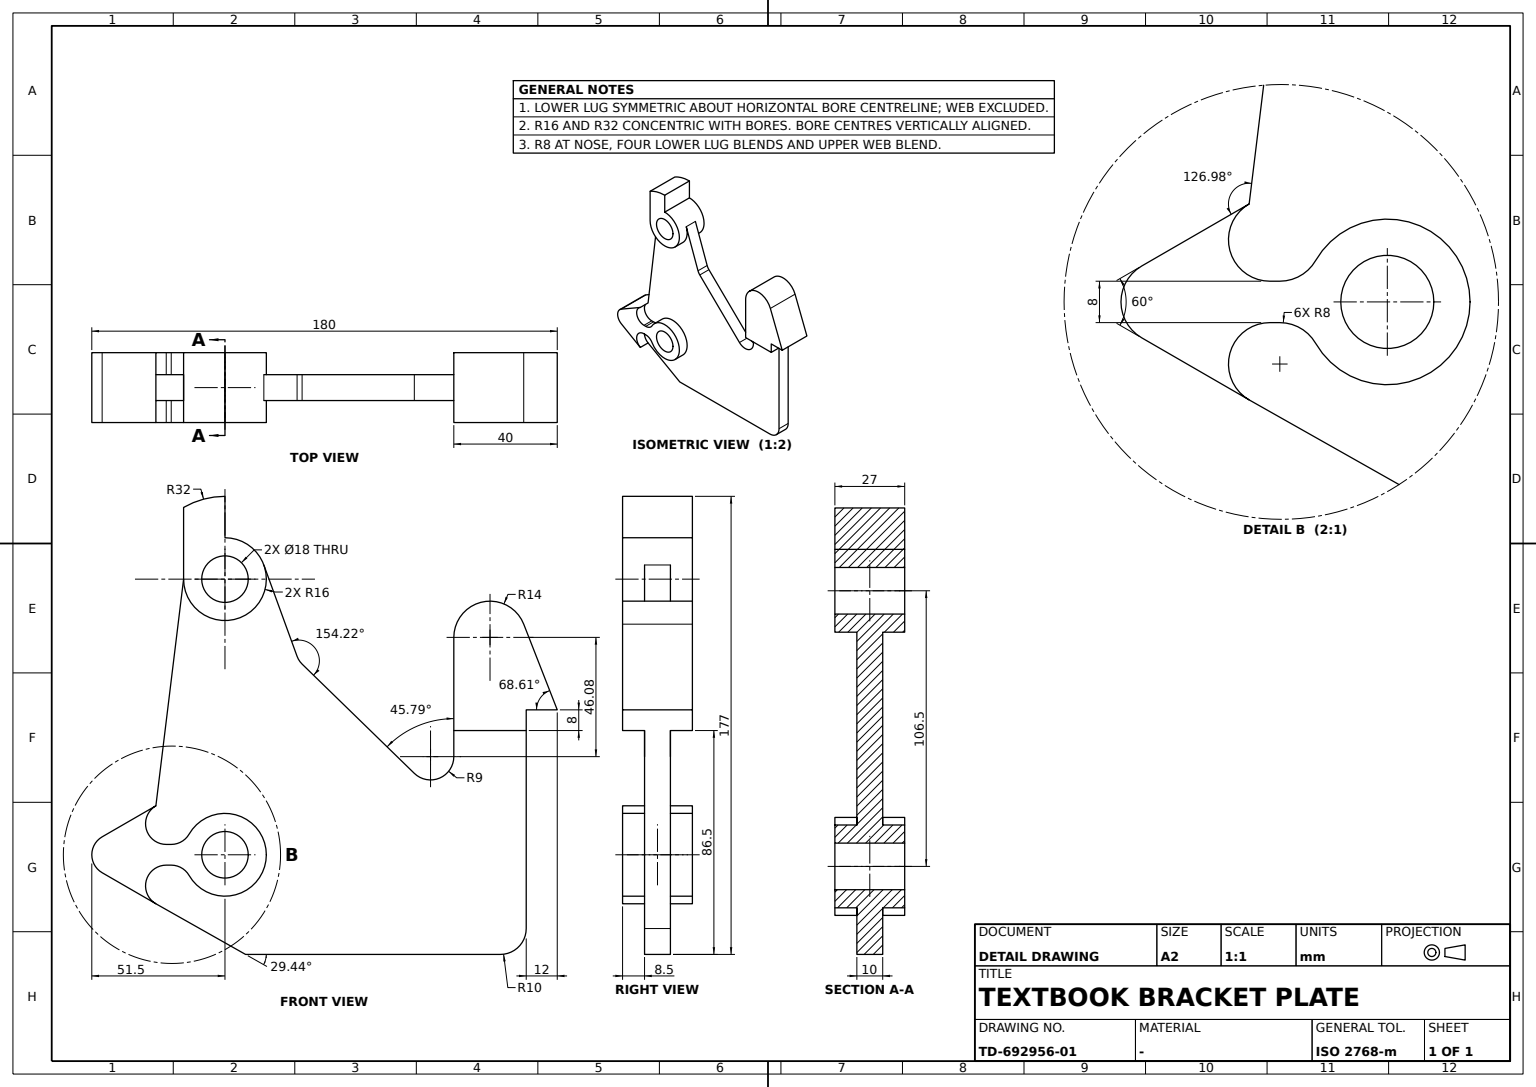
solid
v1 (-13.5,-26.71539,-18.928203)
v2 (-13.5,-22.71539,-4)
e1 v1 v2 CIRCLE(AX(P(-13.5,-22.71539,-12),D(-1,0,0),D(0,1,0)),8)
v3 (-5,-22.71539,-4)
e2 v2 v3 LINE
v4 (-5,-26.71539,-18.928203)
e3 v3 v4 CIRCLE(AX(P(-5,-22.71539,-12),D(1,0,0),D(0,1,0)),8)
e4 v1 v4 LINE
face CYL(AX(P(0,-22.71539,-12),D(-1,0,0),D(0,1,0)),8) rev [e1 e2 e3 -e4]
v5 (-5,106.5,-38.5)
v6 (-5,116.5,-28.5)
e5 v5 v6 CIRCLE(AX(P(-5,106.5,-28.5),D(1,0,0),D(0,1,0)),10)
v7 (5,116.5,-28.5)
e6 v6 v7 LINE
v8 (5,106.5,-38.5)
e7 v8 v7 CIRCLE(AX(P(5,106.5,-28.5),D(1,0,0),D(0,1,0)),10)
e8 v5 v8 LINE
face CYL(AX(P(0,106.5,-28.5),D(-1,0,0),D(0,1,0)),10) [e5 e6 -e7 -e8]
v9 (-5,16,106.5)
v10 (-13.5,16,106.5)
e9 v9 v10 LINE
v11 (-5,-16,106.5)
e10 v9 v11 CIRCLE(AX(P(-5,0,106.5),D(-1,0,0),D(0,1,0)),16)
v12 (-13.5,-16,106.5)
e11 v12 v11 LINE
e12 v12 v10 CIRCLE(AX(P(-13.5,0,106.5),D(1,0,0),D(0,1,0)),16)
face CYL(AX(P(0,0,106.5),D(-1,0,0),D(0,1,0)),16) [-e9 e10 -e11 e12]
v13 (-5,16,0)
v14 (-13.5,16,0)
e13 v13 v14 LINE
v15 (-5,-13.856406,-8)
e14 v13 v15 CIRCLE(AX(P(-5,0,0),D(-1,0,0),D(0,1,0)),16)
v16 (-13.5,-13.856406,-8)
e15 v16 v15 LINE
e16 v16 v14 CIRCLE(AX(P(-13.5,0,0),D(1,0,0),D(0,1,0)),16)
face CYL(AX(P(0,0,0),D(-1,0,0),D(0,1,0)),16) [-e13 e14 -e15 e16]
v17 (-13.5,9,0)
v18 (-13.5,-9,0)
e17 v17 v18 CIRCLE(AX(P(-13.5,0,0),D(1,0,0),D(0,1,0)),9)
v19 (13.5,9,0)
e18 v17 v19 LINE
v20 (13.5,-9,0)
e19 v19 v20 CIRCLE(AX(P(13.5,0,0),D(1,0,0),D(0,1,0)),9)
e20 v18 v20 LINE
face CYL(AX(P(0,0,0),D(-1,0,0),D(0,1,0)),9) rev [-e17 e18 e19 -e20]
v21 (13.5,16,0)
v22 (13.5,-13.856406,8)
e21 v21 v22 CIRCLE(AX(P(13.5,0,0),D(1,0,0),D(0,1,0)),16)
v23 (5,16,0)
e22 v21 v23 LINE
v24 (5,-13.856406,8)
e23 v24 v23 CIRCLE(AX(P(5,0,0),D(-1,0,0),D(0,1,0)),16)
e24 v24 v22 LINE
face CYL(AX(P(0,0,0),D(-1,0,0),D(0,1,0)),16) [-e21 e22 -e23 e24]
e25 v18 v17 CIRCLE(AX(P(-13.5,0,0),D(1,0,0),D(0,1,0)),9)
e26 v20 v19 CIRCLE(AX(P(13.5,0,0),D(1,0,0),D(0,1,0)),9)
face CYL(AX(P(0,0,0),D(-1,0,0),D(0,1,0)),9) rev [-e25 e20 e26 -e18]
v25 (-13.5,-26.71539,18.928203)
v26 (-5,-26.71539,18.928203)
e27 v25 v26 LINE
v27 (-13.5,-47.5,6.928203)
e28 v25 v27 LINE
v28 (13.5,-47.5,6.928203)
e29 v27 v28 LINE
v29 (13.5,-26.71539,18.928203)
e30 v29 v28 LINE
v30 (5,-26.71539,18.928203)
e31 v30 v29 LINE
e32 v26 v30 LINE
face PLANE(AX(P(0,-47.5,6.928203),D(0,0.5,-0.866025404),D(0,0.866025404,0.5))) rev [-e27 e28 e29 -e30 -e31 -e32]
v31 (-13.5,-47.5,-6.928203)
e33 v31 v1 LINE
v32 (5,-26.71539,-18.928203)
e34 v4 v32 LINE
v33 (13.5,-26.71539,-18.928203)
e35 v32 v33 LINE
v34 (13.5,-47.5,-6.928203)
e36 v34 v33 LINE
e37 v31 v34 LINE
face PLANE(AX(P(0,-47.5,-6.928203),D(0,-0.5,-0.866025404),D(0,0.866025404,-0.5))) [e33 e4 e34 e35 -e36 -e37]
v35 (5,-16,106.5)
e38 v35 v30 LINE
e39 v11 v35 LINE
e40 v11 v26 LINE
face PLANE(AX(P(0,-16,106.5),D(0,-0.992596896,0.121455349),D(0,-0.121455349,-0.992596896))) [e32 -e38 -e39 e40]
v36 (13.5,-13.856406,-8)
e41 v36 v21 CIRCLE(AX(P(13.5,0,0),D(1,0,0),D(0,1,0)),16)
v37 (5,-13.856406,-8)
e42 v37 v36 LINE
e43 v23 v37 CIRCLE(AX(P(5,0,0),D(-1,0,0),D(0,1,0)),16)
face CYL(AX(P(0,0,0),D(-1,0,0),D(0,1,0)),16) [-e22 -e41 -e42 -e43]
v38 (-5,116.5,48)
v39 (-5,88.5,48)
e44 v38 v39 LINE
v40 (-13.5,88.5,48)
e45 v40 v39 LINE
v41 (-13.5,116.5,48)
e46 v40 v41 LINE
e47 v41 v38 LINE
face PLANE(AX(P(0,88.5,48),D(0,0,-1),D(0,1,0))) [e44 -e45 e46 e47]
v42 (-5,27.888465,76.67917)
v43 (-5,15.034024,111.975228)
e48 v42 v43 LINE
v44 (5,15.034024,111.975228)
e49 v43 v44 LINE
v45 (5,27.888465,76.67917)
e50 v45 v44 LINE
e51 v42 v45 LINE
face PLANE(AX(P(0,27.888465,76.67917),D(0,0.9396265,0.342201754),D(0,-0.342201754,0.9396265))) [e48 e49 -e50 -e51]
v46 (-13.5,116.5,56)
v47 (13.5,116.5,56)
e52 v46 v47 LINE
v48 (-13.5,128.5,56)
e53 v46 v48 LINE
v49 (13.5,128.5,56)
e54 v48 v49 LINE
e55 v47 v49 LINE
face PLANE(AX(P(0,116.5,56),D(0,0,-1),D(0,1,0))) [-e52 e53 e54 -e55]
v50 (13.5,-20.78461,-4)
e56 v50 v36 CIRCLE(AX(P(13.5,-20.78461,-12),D(-1,0,0),D(0,1,0)),8)
v51 (5,-20.78461,-4)
e57 v51 v50 LINE
e58 v37 v51 CIRCLE(AX(P(5,-20.78461,-12),D(1,0,0),D(0,1,0)),8)
face CYL(AX(P(0,-20.78461,-12),D(-1,0,0),D(0,1,0)),8) rev [-e56 -e57 -e58 e42]
v52 (13.5,16,106.5)
v53 (5,16,106.5)
e59 v52 v53 LINE
v54 (13.5,-16,106.5)
e60 v54 v52 CIRCLE(AX(P(13.5,0,106.5),D(1,0,0),D(0,1,0)),16)
e61 v35 v54 LINE
e62 v53 v35 CIRCLE(AX(P(5,0,106.5),D(-1,0,0),D(0,1,0)),16)
face CYL(AX(P(0,0,106.5),D(-1,0,0),D(0,1,0)),16) [-e59 -e60 -e61 -e62]
v55 (-13.5,9,106.5)
v56 (-13.5,-9,106.5)
e63 v55 v56 CIRCLE(AX(P(-13.5,0,106.5),D(1,0,0),D(0,1,0)),9)
v57 (13.5,9,106.5)
e64 v55 v57 LINE
v58 (13.5,-9,106.5)
e65 v57 v58 CIRCLE(AX(P(13.5,0,106.5),D(1,0,0),D(0,1,0)),9)
e66 v56 v58 LINE
face CYL(AX(P(0,0,106.5),D(-1,0,0),D(0,1,0)),9) rev [-e63 e64 e65 -e66]
v59 (-13.5,115.536088,89.104939)
e67 v48 v59 LINE
v60 (13.5,115.536088,89.104939)
e68 v59 v60 LINE
e69 v49 v60 LINE
face PLANE(AX(P(0,128.5,56),D(0,0.931149161,0.364638506),D(0,-0.364638506,0.931149161))) [e67 e68 -e69 -e54]
v61 (-13.5,88.5,84)
v62 (13.5,88.5,84)
e70 v61 v62 LINE
e71 v60 v62 CIRCLE(AX(P(13.5,102.5,84),D(1,0,0),D(0,1,0)),14)
e72 v59 v61 CIRCLE(AX(P(-13.5,102.5,84),D(1,0,0),D(0,1,0)),14)
face CYL(AX(P(0,102.5,84),D(-1,0,0),D(0,1,0)),14) [e70 -e71 -e68 e72]
e73 v58 v57 CIRCLE(AX(P(13.5,0,106.5),D(1,0,0),D(0,1,0)),9)
v63 (13.5,0,122.5)
e74 v52 v63 CIRCLE(AX(P(13.5,0,106.5),D(1,0,0),D(0,1,0)),16)
v64 (13.5,0,138.5)
e75 v63 v64 LINE
v65 (13.5,-16,134.212813)
e76 v64 v65 CIRCLE(AX(P(13.5,0,106.5),D(1,0,0),D(0,1,0)),32)
e77 v65 v54 LINE
face PLANE(AX(P(13.5,0,0),D(1,0,0),D(0,1,0))) [-e65 -e73] [e60 e74 e75 e76 e77]
v66 (5,-22.71539,-4)
e78 v66 v32 CIRCLE(AX(P(5,-22.71539,-12),D(1,0,0),D(0,1,0)),8)
v67 (13.5,-22.71539,-4)
e79 v66 v67 LINE
e80 v33 v67 CIRCLE(AX(P(13.5,-22.71539,-12),D(-1,0,0),D(0,1,0)),8)
face CYL(AX(P(0,-22.71539,-12),D(-1,0,0),D(0,1,0)),8) rev [-e78 e79 -e80 -e35]
v68 (13.5,88.5,48)
e81 v62 v68 LINE
v69 (13.5,116.5,48)
e82 v68 v69 LINE
e83 v69 v47 LINE
face PLANE(AX(P(13.5,0,0),D(1,0,0),D(0,1,0))) [e71 e81 e82 e83 e55 e69]
v70 (-13.5,-13.856406,8)
v71 (-5,-13.856406,8)
e84 v70 v71 LINE
e85 v71 v13 CIRCLE(AX(P(-5,0,0),D(-1,0,0),D(0,1,0)),16)
e86 v14 v70 CIRCLE(AX(P(-13.5,0,0),D(1,0,0),D(0,1,0)),16)
face CYL(AX(P(0,0,0),D(-1,0,0),D(0,1,0)),16) [e84 e85 e13 e86]
v72 (5,7.959209,-38.5)
e87 v72 v8 LINE
v73 (-5,7.959209,-38.5)
e88 v73 v72 LINE
e89 v73 v5 LINE
face PLANE(AX(P(0,106.5,-38.5),D(0,0,1),D(0,-1,0))) rev [e8 -e87 -e88 e89]
v74 (-13.5,0,138.5)
e90 v74 v64 LINE
v75 (-13.5,-16,134.212813)
e91 v74 v75 CIRCLE(AX(P(-13.5,0,106.5),D(1,0,0),D(0,1,0)),32)
e92 v75 v65 LINE
face CYL(AX(P(0,0,106.5),D(-1,0,0),D(0,1,0)),32) [-e76 -e90 e91 e92]
v76 (5,88.5,37.916968)
v77 (5,73.224396,31.465861)
e93 v76 v77 CIRCLE(AX(P(5,79.5,37.916968),D(-1,0,0),D(0,1,0)),9)
v78 (-5,88.5,37.916968)
e94 v78 v76 LINE
v79 (-5,73.224396,31.465861)
e95 v78 v79 CIRCLE(AX(P(-5,79.5,37.916968),D(-1,0,0),D(0,1,0)),9)
e96 v79 v77 LINE
face CYL(AX(P(0,79.5,37.916968),D(-1,0,0),D(0,1,0)),9) rev [-e93 -e94 e95 e96]
v80 (5,-20.78461,4)
v81 (13.5,-20.78461,4)
e97 v80 v81 LINE
v82 (5,-22.71539,4)
e98 v82 v80 LINE
v83 (13.5,-22.71539,4)
e99 v82 v83 LINE
e100 v81 v83 LINE
face PLANE(AX(P(0,-22.71539,4),D(0,0,-1),D(0,1,0))) rev [-e97 -e98 e99 -e100]
e101 v41 v46 LINE
v84 (5,116.5,48)
e102 v84 v69 LINE
e103 v7 v84 LINE
e104 v6 v38 LINE
face PLANE(AX(P(0,116.5,48),D(0,1,0),D(0,0,1))) [e101 e52 -e83 -e102 -e103 -e6 e104 -e47]
e105 v22 v81 CIRCLE(AX(P(13.5,-20.78461,12),D(-1,0,0),D(0,1,0)),8)
e106 v80 v24 CIRCLE(AX(P(5,-20.78461,12),D(1,0,0),D(0,1,0)),8)
face CYL(AX(P(0,-20.78461,12),D(-1,0,0),D(0,1,0)),8) rev [e97 -e105 -e24 -e106]
v85 (-13.5,-20.78461,-4)
e107 v2 v85 LINE
e108 v27 v31 CIRCLE(AX(P(-13.5,-43.5,0),D(1,0,0),D(0,1,0)),8)
v86 (-13.5,-22.71539,4)
e109 v86 v25 CIRCLE(AX(P(-13.5,-22.71539,12),D(-1,0,0),D(0,1,0)),8)
v87 (-13.5,-20.78461,4)
e110 v87 v86 LINE
e111 v70 v87 CIRCLE(AX(P(-13.5,-20.78461,12),D(-1,0,0),D(0,1,0)),8)
e112 v85 v16 CIRCLE(AX(P(-13.5,-20.78461,-12),D(-1,0,0),D(0,1,0)),8)
face PLANE(AX(P(-13.5,0,0),D(1,0,0),D(0,1,0))) rev [-e107 -e1 -e33 -e108 -e28 -e109 -e110 -e111 -e86 -e16 -e112] [e17 e25]
e113 v61 v40 LINE
e114 v39 v78 LINE
v88 (5,88.5,48)
e115 v88 v76 LINE
e116 v88 v68 LINE
face PLANE(AX(P(0,88.5,48),D(0,1,0),D(0,0,1))) rev [-e70 e113 e45 e114 e94 -e115 e116 -e81]
v89 (5,29.827162,73.682466)
e117 v77 v89 LINE
v90 (-5,29.827162,73.682466)
e118 v79 v90 LINE
e119 v90 v89 LINE
face PLANE(AX(P(0,73.224396,31.465861),D(0,0.697289364,0.716789748),D(0,-0.716789748,0.697289364))) [-e117 -e96 e118 e119]
v91 (-13.5,0,122.5)
e120 v91 v63 LINE
e121 v91 v74 LINE
face PLANE(AX(P(0,0,122.5),D(0,1,0),D(0,0,1))) [-e120 e121 e90 -e75]
v92 (-5,-20.78461,-4)
e122 v85 v92 LINE
e123 v92 v3 LINE
face PLANE(AX(P(0,-22.71539,-4),D(0,0,-1),D(0,1,0))) [e107 e122 e123 -e2]
e124 v56 v55 CIRCLE(AX(P(-13.5,0,106.5),D(1,0,0),D(0,1,0)),9)
face CYL(AX(P(0,0,106.5),D(-1,0,0),D(0,1,0)),9) rev [e66 e73 -e64 -e124]
e125 v28 v34 CIRCLE(AX(P(13.5,-43.5,0),D(1,0,0),D(0,1,0)),8)
face CYL(AX(P(0,-43.5,0),D(-1,0,0),D(0,1,0)),8) [-e29 e108 e37 -e125]
e126 v44 v53 CIRCLE(AX(P(5,0,106.5),D(-1,0,0),D(0,1,0)),16)
e127 v43 v9 CIRCLE(AX(P(-5,0,106.5),D(-1,0,0),D(0,1,0)),16)
e128 v10 v91 CIRCLE(AX(P(-13.5,0,106.5),D(1,0,0),D(0,1,0)),16)
face CYL(AX(P(0,0,106.5),D(-1,0,0),D(0,1,0)),16) [e59 -e126 -e49 e127 e9 e128 e120 -e74]
e129 v30 v82 CIRCLE(AX(P(5,-22.71539,12),D(1,0,0),D(0,1,0)),8)
e130 v83 v29 CIRCLE(AX(P(13.5,-22.71539,12),D(-1,0,0),D(0,1,0)),8)
face CYL(AX(P(0,-22.71539,12),D(-1,0,0),D(0,1,0)),8) rev [-e129 e31 -e130 -e99]
e131 v67 v50 LINE
e132 v51 v66 LINE
face PLANE(AX(P(0,-22.71539,-4),D(0,0,-1),D(0,1,0))) [-e131 -e79 -e132 e57]
face PLANE(AX(P(13.5,0,0),D(1,0,0),D(0,1,0))) [-e19 -e26] [e105 e100 e130 e30 e125 e36 e80 e131 e56 e41 e21]
e133 v75 v12 LINE
face PLANE(AX(P(0,-16,134.212813),D(0,-1,0),D(0,0,-1))) [-e92 e133 e11 e39 e61 -e77]
face PLANE(AX(P(-13.5,0,0),D(1,0,0),D(0,1,0))) rev [-e121 -e128 -e12 -e133 -e91] [e124 e63]
e134 v89 v45 CIRCLE(AX(P(5,35.405477,79.416784),D(-1,0,0),D(0,1,0)),8)
e135 v90 v42 CIRCLE(AX(P(-5,35.405477,79.416784),D(-1,0,0),D(0,1,0)),8)
face CYL(AX(P(0,35.405477,79.416784),D(-1,0,0),D(0,1,0)),8) rev [-e134 -e119 e135 e51]
v93 (-5,-22.71539,4)
v94 (-5,-20.78461,4)
e136 v93 v94 LINE
e137 v87 v94 LINE
e138 v86 v93 LINE
face PLANE(AX(P(0,-22.71539,4),D(0,0,-1),D(0,1,0))) rev [e136 -e137 e110 e138]
e139 v84 v88 LINE
face PLANE(AX(P(0,88.5,48),D(0,0,-1),D(0,1,0))) [-e82 -e116 -e139 e102]
face PLANE(AX(P(-13.5,0,0),D(1,0,0),D(0,1,0))) rev [-e72 -e67 -e53 -e101 -e46 -e113]
e140 v26 v93 CIRCLE(AX(P(-5,-22.71539,12),D(1,0,0),D(0,1,0)),8)
face CYL(AX(P(0,-22.71539,12),D(-1,0,0),D(0,1,0)),8) rev [-e138 e109 e27 e140]
e141 v32 v72 LINE
face PLANE(AX(P(5,0,0),D(1,0,0),D(0,1,0))) [e38 e129 e98 e106 e23 e43 e58 e132 e78 e141 e87 e7 e103 e139 e115 e93 e117 e134 e50 e126 e62]
e142 v4 v73 LINE
e143 v15 v92 CIRCLE(AX(P(-5,-20.78461,-12),D(1,0,0),D(0,1,0)),8)
e144 v94 v71 CIRCLE(AX(P(-5,-20.78461,12),D(1,0,0),D(0,1,0)),8)
face PLANE(AX(P(-5,0,0),D(1,0,0),D(0,1,0))) rev [-e104 -e5 -e89 -e142 -e3 -e123 -e143 -e14 -e85 -e144 -e136 -e140 -e40 -e10 -e127 -e48 -e135 -e118 -e95 -e114 -e44]
face CYL(AX(P(0,-20.78461,12),D(-1,0,0),D(0,1,0)),8) rev [e137 e144 -e84 e111]
face CYL(AX(P(0,-20.78461,-12),D(-1,0,0),D(0,1,0)),8) rev [-e122 e112 e15 e143]
face PLANE(AX(P(0,-26.71539,-18.928203),D(0,-0.491545352,-0.870851978),D(0,0.870851978,-0.491545352))) [e88 -e141 -e34 e142]
